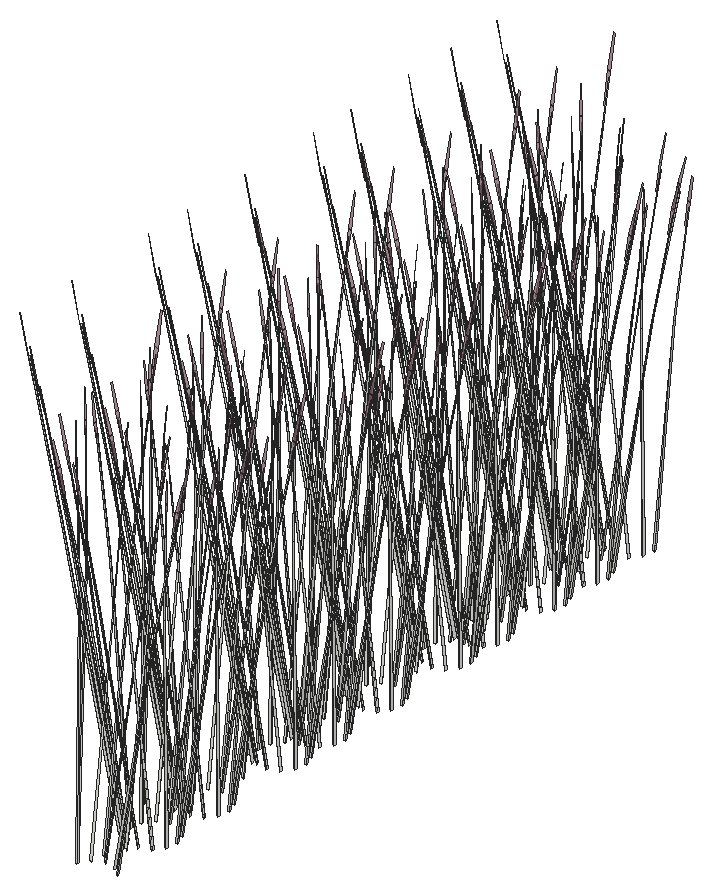
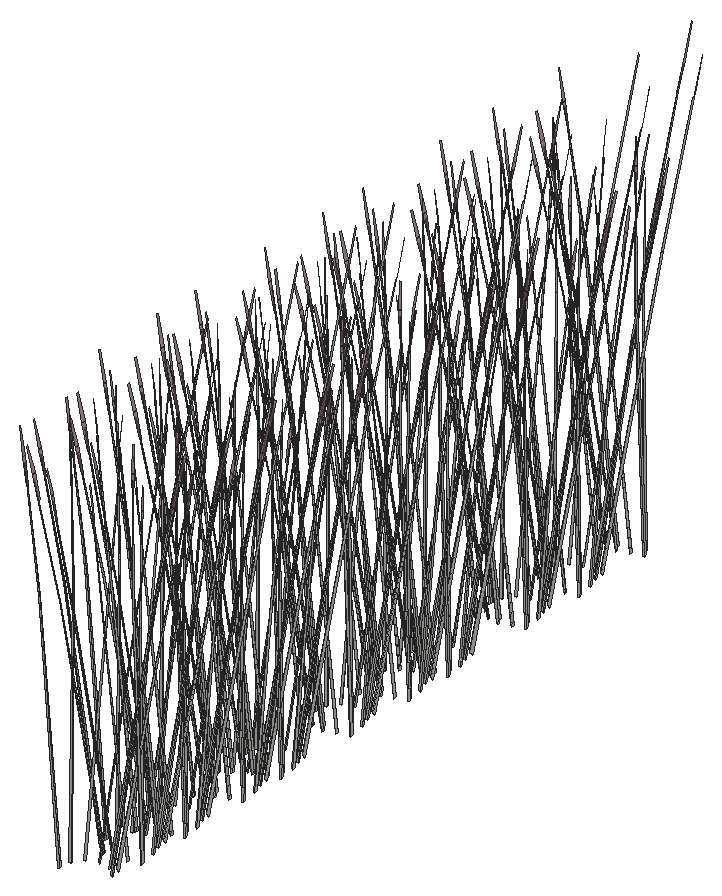
# SketchUp Ruby script. Lengths in inches.
U = 1.inch
M = Sketchup.active_model
def pt(a) = Geom::Point3d.new(a.map { |v| v * U })
def face(e, loops, mat)
  f = e.add_face(loops[0].map { |a| pt(a) })
  loops[1..].each { |l| e.add_face(l.map { |a| pt(a) }).erase! }
  f.material = f.back_material = mat if mat
  f
end
# faces: each face lists its corners as indices into pts; further lists are holes
def faces(e, pts, list, mat = nil) = list.each { |f| face(e, (f[0].is_a?(Array) ? f : [f]).map { |l| l.map { |i| pts[i] } }, mat) }
# xy, xz, yz: faces in a plane at the given z, y or x. An outline is a flat list of corners, or four numbers for a rectangle; further outlines are holes
def ring(l) = l.size == 4 ? [[l[0], l[1]], [l[2], l[1]], [l[2], l[3]], [l[0], l[3]]] : l.each_slice(2).to_a
def flat(e, list, mat, &to3) = list.each { |f| face(e, (f[0].is_a?(Array) ? f : [f]).map { |l| ring(l).map { |u, v| to3.(u, v) } }, mat) }
def xy(e, z, list, mat = nil) = flat(e, list, mat) { |x, y| [x, y, z] }
def xz(e, y, list, mat = nil) = flat(e, list, mat) { |x, z| [x, y, z] }
def yz(e, x, list, mat = nil) = flat(e, list, mat) { |y, z| [x, y, z] }
def lines(e, pts, list) = list.each { |a, b| e.add_line(pt(pts[a]), pt(pts[b])) }
# prism: a flat outline (further loops are holes) pulled along v
def prism(e, loops, v, mat = nil)
  f = face(e, loops, mat); d = Geom::Vector3d.new(v.map { |x| x * U })
  f.pushpull(f.normal.samedirection?(d) ? d.length : -d.length)
end
def box(e, o, s, mat = nil) = prism(e, [[o, [o[0] + s[0], o[1], o[2]], [o[0] + s[0], o[1] + s[1], o[2]], [o[0], o[1] + s[1], o[2]]]], [0, 0, s[2]], mat)
def at(x, y, z, deg = 0) = Geom::Transformation.translation(pt([x, y, z])) * Geom::Transformation.rotation(ORIGIN, Z_AXIS, deg.degrees)
def axes(o, x, y, z) = Geom::Transformation.new([*x, 0, *y, 0, *z, 0, *pt(o).to_a, 1])
def part(name) = M.definitions.add(name)
# library, detail: a bought-in or finely detailed component or shape, given as its bounding box
def library(name, o, s) = part(name).tap { |d| box(d.entities, o, s) }
def detail(e, o, s) = box(e.add_group.entities, o, s)
def put(e, d, t, mat = nil) = e.add_instance(d, t).tap { |i| i.material = mat if mat }
def group(e, t, mat = nil) = e.add_group.tap { |g| g.transformation = t; g.material = mat if mat }.entities
root = M.entities
M.materials.add("LightPink_Translucent").color = [144, 107, 117]
M.materials["LightPink_Translucent"].alpha = 0.75
c1 = part("blade")
p = [[2.15,0.21,22],[0,0.17,0],[0.09,0.45,0],[2.18,0.31,22],[2.29,0.31,22],[0.38,0.45,0],
  [2.48,0.24,33],[2.49,0.24,33],[2.48,0.22,33]]
faces(c1.entities,p,[[0,1,2,3],[4,5,2,3],[6,3,4,7],[8,0,3,6]])
c2 = part("seeds")
p = [[0.3,-0.1,1.38],[-0.01,-0.03,1.59],[-0.01,-0.03,0.03],[0.14,-0.07,-0.07],[0.29,-0.03,3],[0.15,0.01,3.11]]
faces(c2.entities,p,[[0,1,2,3],[1,0,4,5]],"LightPink_Translucent")
c3 = part("blade with seeds")
put(c3.entities,c1,at(0,0,0))
put(c3.entities,c2,axes([2.4,0.25,30.99],[1.5799,-0.05474,1.17369],[-0.12525,1.92788,0.29478],[-0.07173,-0.02425,1.56792]))
put(root,c3,axes([428.4,426.56,154.3],[0.45651,-0.12123,0.45419],[0.07923,0.47555,0.3745],[-0.10736,-0.14016,0.93983]))
put(root,c3,axes([430.36,423.77,154.27],[-0.23317,-0.29531,0.29918],[0.26625,-0.27955,-0.38624],[0.13527,0.04253,0.73904]))
put(root,c3,axes([429.43,426.95,154.27],[-0.12355,0.36271,0.29918],[-0.36044,-0.10579,-0.38624],[-0.03305,-0.14603,0.73904]))
put(root,c3,axes([427.52,423.16,154.27],[0.35672,-0.06741,0.29918],[0.09419,0.38534,-0.38624],[-0.10222,0.1035,0.73904]))
put(root,c3,axes([430.21,427.36,154.27],[-0.27728,0.24833,0.29918],[-0.26248,-0.28355,-0.38624],[0.03994,-0.14407,0.73904]))
put(root,c3,axes([426.71,424.26,154.77],[0.36162,0.1259,-0.05481],[-0.11124,0.3875,-0.2485],[-0.05915,0.05883,0.81966]))
put(root,c3,axes([428.56,427.01,154.27],[0.06329,0.37991,0.29918],[-0.36182,0.10032,-0.38624],[-0.09718,-0.10887,0.73904]))
put(root,c3,axes([427.48,427.26,154.3],[0.33843,-0.34808,0.45419],[0.29188,0.36965,0.3745],[-0.15878,-0.06421,0.93983]))
put(root,c3,axes([429.64,424.28,154.27],[-0.06329,-0.37991,0.29918],[0.36182,-0.10032,-0.38624],[0.09718,0.10887,0.73904]))
put(root,c3,axes([428,423.93,154.27],[0.27728,-0.24833,0.29918],[0.26248,0.28355,-0.38624],[-0.03994,0.14407,0.73904]))
put(root,c3,axes([430.6875,428.13,154.27],[-0.35672,0.06741,0.29918],[-0.09419,-0.38534,-0.38624],[0.10222,-0.1035,0.73904]))
put(root,c3,axes([428.78,424.34,154.27],[0.12355,-0.36271,0.29918],[0.36044,0.10579,-0.38624],[0.03305,0.14603,0.73904]))
put(root,c3,axes([429.26,425.63,154.77],[0.28319,-0.27058,-0.05481],[0.25948,0.29635,-0.2485],[0.01827,0.08397,0.81966]))
put(root,c3,axes([427.84,427.53,154.27],[0.23317,0.29531,0.29918],[-0.26625,0.27955,-0.38624],[-0.13527,-0.04253,0.73904]))
put(root,c3,axes([428.77,424.64,154.28],[-0.4038,-0.12331,0.45013],[0.13808,-0.40538,0.37115],[0.02427,0.15942,0.93144]))
put(root,c3,axes([430.75,429.05,154.27],[-0.34057,-0.13158,0.29918],[0.09933,-0.38387,-0.38624],[0.13712,-0.0352,0.73904]))
put(root,c3,axes([428.4,431.48,154.3],[0.45651,-0.12123,0.45419],[0.07923,0.47555,0.3745],[-0.10736,-0.14016,0.93983]))
put(root,c3,axes([427.46,428.35,154.27],[0.34057,0.13158,0.29918],[-0.09933,0.38387,-0.38624],[-0.13712,0.0352,0.73904]))
put(root,c3,axes([429.43,431.87,154.27],[-0.12355,0.36271,0.29918],[-0.36044,-0.10579,-0.38624],[-0.03305,-0.14603,0.73904]))
put(root,c3,axes([430.21,432.27,154.27],[-0.27728,0.24833,0.29918],[-0.26248,-0.28355,-0.38624],[0.03994,-0.14407,0.73904]))
put(root,c3,axes([430.36,429.88,154.27],[-0.23317,-0.29531,0.29918],[0.26625,-0.27955,-0.38624],[0.13527,0.04253,0.73904]))
put(root,c3,axes([428.56,431.93,154.27],[0.06329,0.37991,0.29918],[-0.36182,0.10032,-0.38624],[-0.09718,-0.10887,0.73904]))
put(root,c3,axes([427.48,432.17,154.3],[0.33843,-0.34808,0.45419],[0.29188,0.36965,0.3745],[-0.15878,-0.06421,0.93983]))
put(root,c3,axes([427.52,429.27,154.27],[0.35672,-0.06741,0.29918],[0.09419,0.38534,-0.38624],[-0.10222,0.1035,0.73904]))
put(root,c3,axes([430.6875,433.04,154.27],[-0.35672,0.06741,0.29918],[-0.09419,-0.38534,-0.38624],[0.10222,-0.1035,0.73904]))
put(root,c3,axes([426.71,430.37,154.77],[0.36162,0.1259,-0.05481],[-0.11124,0.3875,-0.2485],[-0.05915,0.05883,0.81966]))
put(root,c3,axes([429.64,430.39,154.27],[-0.06329,-0.37991,0.29918],[0.36182,-0.10032,-0.38624],[0.09718,0.10887,0.73904]))
put(root,c3,axes([427.84,432.4375,154.27],[0.23317,0.29531,0.29918],[-0.26625,0.27955,-0.38624],[-0.13527,-0.04253,0.73904]))
put(root,c3,axes([428,430.04,154.27],[0.27728,-0.24833,0.29918],[0.26248,0.28355,-0.38624],[-0.03994,0.14407,0.73904]))
put(root,c3,axes([428.78,430.45,154.27],[0.12355,-0.36271,0.29918],[0.36044,0.10579,-0.38624],[0.03305,0.14603,0.73904]))
put(root,c3,axes([429.26,431.74,154.77],[0.28319,-0.27058,-0.05481],[0.25948,0.29635,-0.2485],[0.01827,0.08397,0.81966]))
put(root,c3,axes([430.75,433.96,154.27],[-0.34057,-0.13158,0.29918],[0.09933,-0.38387,-0.38624],[0.13712,-0.0352,0.73904]))
put(root,c3,axes([428.77,430.75,154.28],[-0.4038,-0.12331,0.45013],[0.13808,-0.40538,0.37115],[0.02427,0.15942,0.93144]))
put(root,c3,axes([427.46,433.27,154.27],[0.34057,0.13158,0.29918],[-0.09933,0.38387,-0.38624],[-0.13712,0.0352,0.73904]))
put(root,c3,axes([430.36,434.79,154.27],[-0.23317,-0.29531,0.29918],[0.26625,-0.27955,-0.38624],[0.13527,0.04253,0.73904]))
put(root,c3,axes([427.52,434.1875,154.27],[0.35672,-0.06741,0.29918],[0.09419,0.38534,-0.38624],[-0.10222,0.1035,0.73904]))
put(root,c3,axes([428.4,438.73,154.3],[0.45651,-0.12123,0.45419],[0.07923,0.47555,0.3745],[-0.10736,-0.14016,0.93983]))
put(root,c3,axes([426.71,435.28,154.77],[0.36162,0.1259,-0.05481],[-0.11124,0.3875,-0.2485],[-0.05915,0.05883,0.81966]))
put(root,c3,axes([429.64,435.3,154.27],[-0.06329,-0.37991,0.29918],[0.36182,-0.10032,-0.38624],[0.09718,0.10887,0.73904]))
put(root,c3,axes([429.43,439.12,154.27],[-0.12355,0.36271,0.29918],[-0.36044,-0.10579,-0.38624],[-0.03305,-0.14603,0.73904]))
put(root,c3,axes([430.21,439.53,154.27],[-0.27728,0.24833,0.29918],[-0.26248,-0.28355,-0.38624],[0.03994,-0.14407,0.73904]))
put(root,c3,axes([428,434.96,154.27],[0.27728,-0.24833,0.29918],[0.26248,0.28355,-0.38624],[-0.03994,0.14407,0.73904]))
put(root,c3,axes([428.78,435.36,154.27],[0.12355,-0.36271,0.29918],[0.36044,0.10579,-0.38624],[0.03305,0.14603,0.73904]))
put(root,c3,axes([428.56,439.18,154.27],[0.06329,0.37991,0.29918],[-0.36182,0.10032,-0.38624],[-0.09718,-0.10887,0.73904]))
put(root,c3,axes([427.48,439.43,154.3],[0.33843,-0.34808,0.45419],[0.29188,0.36965,0.3745],[-0.15878,-0.06421,0.93983]))
put(root,c3,axes([429.26,436.66,154.77],[0.28319,-0.27058,-0.05481],[0.25948,0.29635,-0.2485],[0.01827,0.08397,0.81966]))
put(root,c3,axes([428.77,435.66,154.28],[-0.4038,-0.12331,0.45013],[0.13808,-0.40538,0.37115],[0.02427,0.15942,0.93144]))
put(root,c3,axes([430.6875,440.3,154.27],[-0.35672,0.06741,0.29918],[-0.09419,-0.38534,-0.38624],[0.10222,-0.1035,0.73904]))
put(root,c3,axes([427.84,439.69,154.27],[0.23317,0.29531,0.29918],[-0.26625,0.27955,-0.38624],[-0.13527,-0.04253,0.73904]))
put(root,c3,axes([428.4,442.43,154.3],[0.45651,-0.12123,0.45419],[0.07923,0.47555,0.3745],[-0.10736,-0.14016,0.93983]))
put(root,c3,axes([430.75,441.22,154.27],[-0.34057,-0.13158,0.29918],[0.09933,-0.38387,-0.38624],[0.13712,-0.0352,0.73904]))
put(root,c3,axes([429.43,442.8125,154.27],[-0.12355,0.36271,0.29918],[-0.36044,-0.10579,-0.38624],[-0.03305,-0.14603,0.73904]))
put(root,c3,axes([430.21,443.22,154.27],[-0.27728,0.24833,0.29918],[-0.26248,-0.28355,-0.38624],[0.03994,-0.14407,0.73904]))
put(root,c3,axes([427.46,440.52,154.27],[0.34057,0.13158,0.29918],[-0.09933,0.38387,-0.38624],[-0.13712,0.0352,0.73904]))
put(root,c3,axes([428.56,442.87,154.27],[0.06329,0.37991,0.29918],[-0.36182,0.10032,-0.38624],[-0.09718,-0.10887,0.73904]))
put(root,c3,axes([427.48,443.12,154.3],[0.33843,-0.34808,0.45419],[0.29188,0.36965,0.3745],[-0.15878,-0.06421,0.93983]))
put(root,c3,axes([430.6875,443.99,154.27],[-0.35672,0.06741,0.29918],[-0.09419,-0.38534,-0.38624],[0.10222,-0.1035,0.73904]))
put(root,c3,axes([430.36,442.05,154.27],[-0.23317,-0.29531,0.29918],[0.26625,-0.27955,-0.38624],[0.13527,0.04253,0.73904]))
put(root,c3,axes([427.84,443.39,154.27],[0.23317,0.29531,0.29918],[-0.26625,0.27955,-0.38624],[-0.13527,-0.04253,0.73904]))
put(root,c3,axes([427.52,441.44,154.27],[0.35672,-0.06741,0.29918],[0.09419,0.38534,-0.38624],[-0.10222,0.1035,0.73904]))
put(root,c3,axes([426.71,442.54,154.77],[0.36162,0.1259,-0.05481],[-0.11124,0.3875,-0.2485],[-0.05915,0.05883,0.81966]))
put(root,c3,axes([429.64,442.56,154.27],[-0.06329,-0.37991,0.29918],[0.36182,-0.10032,-0.38624],[0.09718,0.10887,0.73904]))
put(root,c3,axes([430.75,444.91,154.27],[-0.34057,-0.13158,0.29918],[0.09933,-0.38387,-0.38624],[0.13712,-0.0352,0.73904]))
put(root,c3,axes([428,442.21,154.27],[0.27728,-0.24833,0.29918],[0.26248,0.28355,-0.38624],[-0.03994,0.14407,0.73904]))
put(root,c3,axes([428.78,442.62,154.27],[0.12355,-0.36271,0.29918],[0.36044,0.10579,-0.38624],[0.03305,0.14603,0.73904]))
put(root,c3,axes([429.26,443.91,154.77],[0.28319,-0.27058,-0.05481],[0.25948,0.29635,-0.2485],[0.01827,0.08397,0.81966]))
put(root,c3,axes([427.46,444.21,154.27],[0.34057,0.13158,0.29918],[-0.09933,0.38387,-0.38624],[-0.13712,0.0352,0.73904]))
put(root,c3,axes([428.4,447.85,154.3],[0.45651,-0.12123,0.45419],[0.07923,0.47555,0.3745],[-0.10736,-0.14016,0.93983]))
put(root,c3,axes([428.77,442.92,154.28],[-0.4038,-0.12331,0.45013],[0.13808,-0.40538,0.37115],[0.02427,0.15942,0.93144]))
put(root,c3,axes([430.36,445.74,154.27],[-0.23317,-0.29531,0.29918],[0.26625,-0.27955,-0.38624],[0.13527,0.04253,0.73904]))
put(root,c3,axes([429.43,448.23,154.27],[-0.12355,0.36271,0.29918],[-0.36044,-0.10579,-0.38624],[-0.03305,-0.14603,0.73904]))
put(root,c3,axes([430.21,448.64,154.27],[-0.27728,0.24833,0.29918],[-0.26248,-0.28355,-0.38624],[0.03994,-0.14407,0.73904]))
put(root,c3,axes([428.56,448.29,154.27],[0.06329,0.37991,0.29918],[-0.36182,0.10032,-0.38624],[-0.09718,-0.10887,0.73904]))
put(root,c3,axes([427.48,448.54,154.3],[0.33843,-0.34808,0.45419],[0.29188,0.36965,0.3745],[-0.15878,-0.06421,0.93983]))
put(root,c3,axes([427.52,445.13,154.27],[0.35672,-0.06741,0.29918],[0.09419,0.38534,-0.38624],[-0.10222,0.1035,0.73904]))
put(root,c3,axes([430.6875,449.41,154.27],[-0.35672,0.06741,0.29918],[-0.09419,-0.38534,-0.38624],[0.10222,-0.1035,0.73904]))
put(root,c3,axes([426.71,446.23,154.77],[0.36162,0.1259,-0.05481],[-0.11124,0.3875,-0.2485],[-0.05915,0.05883,0.81966]))
put(root,c3,axes([429.64,446.25,154.27],[-0.06329,-0.37991,0.29918],[0.36182,-0.10032,-0.38624],[0.09718,0.10887,0.73904]))
put(root,c3,axes([428,445.9,154.27],[0.27728,-0.24833,0.29918],[0.26248,0.28355,-0.38624],[-0.03994,0.14407,0.73904]))
put(root,c3,axes([428.78,446.3125,154.27],[0.12355,-0.36271,0.29918],[0.36044,0.10579,-0.38624],[0.03305,0.14603,0.73904]))
put(root,c3,axes([427.84,448.81,154.27],[0.23317,0.29531,0.29918],[-0.26625,0.27955,-0.38624],[-0.13527,-0.04253,0.73904]))
put(root,c3,axes([429.26,447.6,154.77],[0.28319,-0.27058,-0.05481],[0.25948,0.29635,-0.2485],[0.01827,0.08397,0.81966]))
put(root,c3,axes([428.77,446.61,154.28],[-0.4038,-0.12331,0.45013],[0.13808,-0.40538,0.37115],[0.02427,0.15942,0.93144]))
put(root,c3,axes([430.75,450.33,154.27],[-0.34057,-0.13158,0.29918],[0.09933,-0.38387,-0.38624],[0.13712,-0.0352,0.73904]))
put(root,c3,axes([427.46,449.64,154.27],[0.34057,0.13158,0.29918],[-0.09933,0.38387,-0.38624],[-0.13712,0.0352,0.73904]))
put(root,c3,axes([430.36,451.16,154.27],[-0.23317,-0.29531,0.29918],[0.26625,-0.27955,-0.38624],[0.13527,0.04253,0.73904]))
put(root,c3,axes([428.4,454.33,154.3],[0.45651,-0.12123,0.45419],[0.07923,0.47555,0.3745],[-0.10736,-0.14016,0.93983]))
put(root,c3,axes([427.52,450.56,154.27],[0.35672,-0.06741,0.29918],[0.09419,0.38534,-0.38624],[-0.10222,0.1035,0.73904]))
put(root,c3,axes([429.43,454.72,154.27],[-0.12355,0.36271,0.29918],[-0.36044,-0.10579,-0.38624],[-0.03305,-0.14603,0.73904]))
put(root,c3,axes([430.21,455.125,154.27],[-0.27728,0.24833,0.29918],[-0.26248,-0.28355,-0.38624],[0.03994,-0.14407,0.73904]))
put(root,c3,axes([426.71,451.65,154.77],[0.36162,0.1259,-0.05481],[-0.11124,0.3875,-0.2485],[-0.05915,0.05883,0.81966]))
put(root,c3,axes([429.64,451.67,154.27],[-0.06329,-0.37991,0.29918],[0.36182,-0.10032,-0.38624],[0.09718,0.10887,0.73904]))
put(root,c3,axes([428.56,454.78,154.27],[0.06329,0.37991,0.29918],[-0.36182,0.10032,-0.38624],[-0.09718,-0.10887,0.73904]))
put(root,c3,axes([427.48,455.02,154.3],[0.33843,-0.34808,0.45419],[0.29188,0.36965,0.3745],[-0.15878,-0.06421,0.93983]))
put(root,c3,axes([428,451.32,154.27],[0.27728,-0.24833,0.29918],[0.26248,0.28355,-0.38624],[-0.03994,0.14407,0.73904]))
put(root,c3,axes([428.78,451.73,154.27],[0.12355,-0.36271,0.29918],[0.36044,0.10579,-0.38624],[0.03305,0.14603,0.73904]))
put(root,c3,axes([430.6875,455.89,154.27],[-0.35672,0.06741,0.29918],[-0.09419,-0.38534,-0.38624],[0.10222,-0.1035,0.73904]))
put(root,c3,axes([429.26,453.03,154.77],[0.28319,-0.27058,-0.05481],[0.25948,0.29635,-0.2485],[0.01827,0.08397,0.81966]))
put(root,c3,axes([428.77,452.03,154.28],[-0.4038,-0.12331,0.45013],[0.13808,-0.40538,0.37115],[0.02427,0.15942,0.93144]))
put(root,c3,axes([427.84,455.29,154.27],[0.23317,0.29531,0.29918],[-0.26625,0.27955,-0.38624],[-0.13527,-0.04253,0.73904]))
put(root,c3,axes([428.4,457.875,154.3],[0.45651,-0.12123,0.45419],[0.07923,0.47555,0.3745],[-0.10736,-0.14016,0.93983]))
put(root,c3,axes([430.75,456.8125,154.27],[-0.34057,-0.13158,0.29918],[0.09933,-0.38387,-0.38624],[0.13712,-0.0352,0.73904]))
put(root,c3,axes([429.43,458.26,154.27],[-0.12355,0.36271,0.29918],[-0.36044,-0.10579,-0.38624],[-0.03305,-0.14603,0.73904]))
put(root,c3,axes([430.21,458.67,154.27],[-0.27728,0.24833,0.29918],[-0.26248,-0.28355,-0.38624],[0.03994,-0.14407,0.73904]))
put(root,c3,axes([428.56,458.32,154.27],[0.06329,0.37991,0.29918],[-0.36182,0.10032,-0.38624],[-0.09718,-0.10887,0.73904]))
put(root,c3,axes([427.48,458.57,154.3],[0.33843,-0.34808,0.45419],[0.29188,0.36965,0.3745],[-0.15878,-0.06421,0.93983]))
put(root,c3,axes([427.46,456.12,154.27],[0.34057,0.13158,0.29918],[-0.09933,0.38387,-0.38624],[-0.13712,0.0352,0.73904]))
put(root,c3,axes([430.6875,459.44,154.27],[-0.35672,0.06741,0.29918],[-0.09419,-0.38534,-0.38624],[0.10222,-0.1035,0.73904]))
put(root,c3,axes([430.36,457.64,154.27],[-0.23317,-0.29531,0.29918],[0.26625,-0.27955,-0.38624],[0.13527,0.04253,0.73904]))
put(root,c3,axes([427.84,458.84,154.27],[0.23317,0.29531,0.29918],[-0.26625,0.27955,-0.38624],[-0.13527,-0.04253,0.73904]))
put(root,c3,axes([427.52,457.04,154.27],[0.35672,-0.06741,0.29918],[0.09419,0.38534,-0.38624],[-0.10222,0.1035,0.73904]))
put(root,c3,axes([430.75,460.36,154.27],[-0.34057,-0.13158,0.29918],[0.09933,-0.38387,-0.38624],[0.13712,-0.0352,0.73904]))
put(root,c3,axes([426.71,458.13,154.77],[0.36162,0.1259,-0.05481],[-0.11124,0.3875,-0.2485],[-0.05915,0.05883,0.81966]))
put(root,c3,axes([429.64,458.16,154.27],[-0.06329,-0.37991,0.29918],[0.36182,-0.10032,-0.38624],[0.09718,0.10887,0.73904]))
put(root,c3,axes([428,457.81,154.27],[0.27728,-0.24833,0.29918],[0.26248,0.28355,-0.38624],[-0.03994,0.14407,0.73904]))
put(root,c3,axes([428.78,458.22,154.27],[0.12355,-0.36271,0.29918],[0.36044,0.10579,-0.38624],[0.03305,0.14603,0.73904]))
put(root,c3,axes([427.46,459.67,154.27],[0.34057,0.13158,0.29918],[-0.09933,0.38387,-0.38624],[-0.13712,0.0352,0.73904]))
put(root,c3,axes([428.4,463.28,154.3],[0.45651,-0.12123,0.45419],[0.07923,0.47555,0.3745],[-0.10736,-0.14016,0.93983]))
put(root,c3,axes([429.26,459.51,154.77],[0.28319,-0.27058,-0.05481],[0.25948,0.29635,-0.2485],[0.01827,0.08397,0.81966]))
put(root,c3,axes([428.77,458.51,154.28],[-0.4038,-0.12331,0.45013],[0.13808,-0.40538,0.37115],[0.02427,0.15942,0.93144]))
put(root,c3,axes([430.36,461.19,154.27],[-0.23317,-0.29531,0.29918],[0.26625,-0.27955,-0.38624],[0.13527,0.04253,0.73904]))
put(root,c3,axes([429.43,463.67,154.27],[-0.12355,0.36271,0.29918],[-0.36044,-0.10579,-0.38624],[-0.03305,-0.14603,0.73904]))
put(root,c3,axes([430.21,464.08,154.27],[-0.27728,0.24833,0.29918],[-0.26248,-0.28355,-0.38624],[0.03994,-0.14407,0.73904]))
put(root,c3,axes([428.56,463.73,154.27],[0.06329,0.37991,0.29918],[-0.36182,0.10032,-0.38624],[-0.09718,-0.10887,0.73904]))
put(root,c3,axes([427.48,463.97,154.3],[0.33843,-0.34808,0.45419],[0.29188,0.36965,0.3745],[-0.15878,-0.06421,0.93983]))
put(root,c3,axes([427.52,460.59,154.27],[0.35672,-0.06741,0.29918],[0.09419,0.38534,-0.38624],[-0.10222,0.1035,0.73904]))
put(root,c3,axes([430.6875,464.84,154.27],[-0.35672,0.06741,0.29918],[-0.09419,-0.38534,-0.38624],[0.10222,-0.1035,0.73904]))
put(root,c3,axes([426.71,461.68,154.77],[0.36162,0.1259,-0.05481],[-0.11124,0.3875,-0.2485],[-0.05915,0.05883,0.81966]))
put(root,c3,axes([429.64,461.7,154.27],[-0.06329,-0.37991,0.29918],[0.36182,-0.10032,-0.38624],[0.09718,0.10887,0.73904]))
put(root,c3,axes([428,461.35,154.27],[0.27728,-0.24833,0.29918],[0.26248,0.28355,-0.38624],[-0.03994,0.14407,0.73904]))
put(root,c3,axes([428.78,461.76,154.27],[0.12355,-0.36271,0.29918],[0.36044,0.10579,-0.38624],[0.03305,0.14603,0.73904]))
put(root,c3,axes([427.84,464.24,154.27],[0.23317,0.29531,0.29918],[-0.26625,0.27955,-0.38624],[-0.13527,-0.04253,0.73904]))
put(root,c3,axes([429.26,463.06,154.77],[0.28319,-0.27058,-0.05481],[0.25948,0.29635,-0.2485],[0.01827,0.08397,0.81966]))
put(root,c3,axes([428.77,462.0625,154.28],[-0.4038,-0.12331,0.45013],[0.13808,-0.40538,0.37115],[0.02427,0.15942,0.93144]))
put(root,c3,axes([428.4,467.33,154.3],[0.45651,-0.12123,0.45419],[0.07923,0.47555,0.3745],[-0.10736,-0.14016,0.93983]))
put(root,c3,axes([430.75,465.76,154.27],[-0.34057,-0.13158,0.29918],[0.09933,-0.38387,-0.38624],[0.13712,-0.0352,0.73904]))
put(root,c3,axes([429.43,467.72,154.27],[-0.12355,0.36271,0.29918],[-0.36044,-0.10579,-0.38624],[-0.03305,-0.14603,0.73904]))
put(root,c3,axes([430.21,468.13,154.27],[-0.27728,0.24833,0.29918],[-0.26248,-0.28355,-0.38624],[0.03994,-0.14407,0.73904]))
put(root,c3,axes([427.46,465.07,154.27],[0.34057,0.13158,0.29918],[-0.09933,0.38387,-0.38624],[-0.13712,0.0352,0.73904]))
put(root,c3,axes([428.56,467.78,154.27],[0.06329,0.37991,0.29918],[-0.36182,0.10032,-0.38624],[-0.09718,-0.10887,0.73904]))
put(root,c3,axes([427.48,468.03,154.3],[0.33843,-0.34808,0.45419],[0.29188,0.36965,0.3745],[-0.15878,-0.06421,0.93983]))
put(root,c3,axes([430.36,466.59,154.27],[-0.23317,-0.29531,0.29918],[0.26625,-0.27955,-0.38624],[0.13527,0.04253,0.73904]))
put(root,c3,axes([430.6875,468.9,154.27],[-0.35672,0.06741,0.29918],[-0.09419,-0.38534,-0.38624],[0.10222,-0.1035,0.73904]))
put(root,c3,axes([427.52,465.99,154.27],[0.35672,-0.06741,0.29918],[0.09419,0.38534,-0.38624],[-0.10222,0.1035,0.73904]))
put(root,c3,axes([427.84,468.29,154.27],[0.23317,0.29531,0.29918],[-0.26625,0.27955,-0.38624],[-0.13527,-0.04253,0.73904]))
put(root,c3,axes([426.71,467.08,154.77],[0.36162,0.1259,-0.05481],[-0.11124,0.3875,-0.2485],[-0.05915,0.05883,0.81966]))
put(root,c3,axes([429.64,467.11,154.27],[-0.06329,-0.37991,0.29918],[0.36182,-0.10032,-0.38624],[0.09718,0.10887,0.73904]))
put(root,c3,axes([430.75,469.82,154.27],[-0.34057,-0.13158,0.29918],[0.09933,-0.38387,-0.38624],[0.13712,-0.0352,0.73904]))
put(root,c3,axes([428.4,471.66,154.3],[0.45651,-0.12123,0.45419],[0.07923,0.47555,0.3745],[-0.10736,-0.14016,0.93983]))
put(root,c3,axes([428,466.76,154.27],[0.27728,-0.24833,0.29918],[0.26248,0.28355,-0.38624],[-0.03994,0.14407,0.73904]))
put(root,c3,axes([428.78,467.17,154.27],[0.12355,-0.36271,0.29918],[0.36044,0.10579,-0.38624],[0.03305,0.14603,0.73904]))
put(root,c3,axes([429.26,468.46,154.77],[0.28319,-0.27058,-0.05481],[0.25948,0.29635,-0.2485],[0.01827,0.08397,0.81966]))
put(root,c3,axes([429.43,472.05,154.27],[-0.12355,0.36271,0.29918],[-0.36044,-0.10579,-0.38624],[-0.03305,-0.14603,0.73904]))
put(root,c3,axes([427.46,469.12,154.27],[0.34057,0.13158,0.29918],[-0.09933,0.38387,-0.38624],[-0.13712,0.0352,0.73904]))
put(root,c3,axes([428.77,467.46,154.28],[-0.4038,-0.12331,0.45013],[0.13808,-0.40538,0.37115],[0.02427,0.15942,0.93144]))
put(root,c3,axes([430.21,472.45,154.27],[-0.27728,0.24833,0.29918],[-0.26248,-0.28355,-0.38624],[0.03994,-0.14407,0.73904]))
put(root,c3,axes([428.56,472.11,154.27],[0.06329,0.37991,0.29918],[-0.36182,0.10032,-0.38624],[-0.09718,-0.10887,0.73904]))
put(root,c3,axes([427.48,472.35,154.3],[0.33843,-0.34808,0.45419],[0.29188,0.36965,0.3745],[-0.15878,-0.06421,0.93983]))
put(root,c3,axes([430.36,470.65,154.27],[-0.23317,-0.29531,0.29918],[0.26625,-0.27955,-0.38624],[0.13527,0.04253,0.73904]))
put(root,c3,axes([430.6875,473.22,154.27],[-0.35672,0.06741,0.29918],[-0.09419,-0.38534,-0.38624],[0.10222,-0.1035,0.73904]))
put(root,c3,axes([427.52,470.04,154.27],[0.35672,-0.06741,0.29918],[0.09419,0.38534,-0.38624],[-0.10222,0.1035,0.73904]))
put(root,c3,axes([427.84,472.62,154.27],[0.23317,0.29531,0.29918],[-0.26625,0.27955,-0.38624],[-0.13527,-0.04253,0.73904]))
put(root,c3,axes([426.71,471.14,154.77],[0.36162,0.1259,-0.05481],[-0.11124,0.3875,-0.2485],[-0.05915,0.05883,0.81966]))
put(root,c3,axes([429.64,471.16,154.27],[-0.06329,-0.37991,0.29918],[0.36182,-0.10032,-0.38624],[0.09718,0.10887,0.73904]))
put(root,c3,axes([428,470.81,154.27],[0.27728,-0.24833,0.29918],[0.26248,0.28355,-0.38624],[-0.03994,0.14407,0.73904]))
put(root,c3,axes([430.75,474.14,154.27],[-0.34057,-0.13158,0.29918],[0.09933,-0.38387,-0.38624],[0.13712,-0.0352,0.73904]))
put(root,c3,axes([428.78,471.22,154.27],[0.12355,-0.36271,0.29918],[0.36044,0.10579,-0.38624],[0.03305,0.14603,0.73904]))
